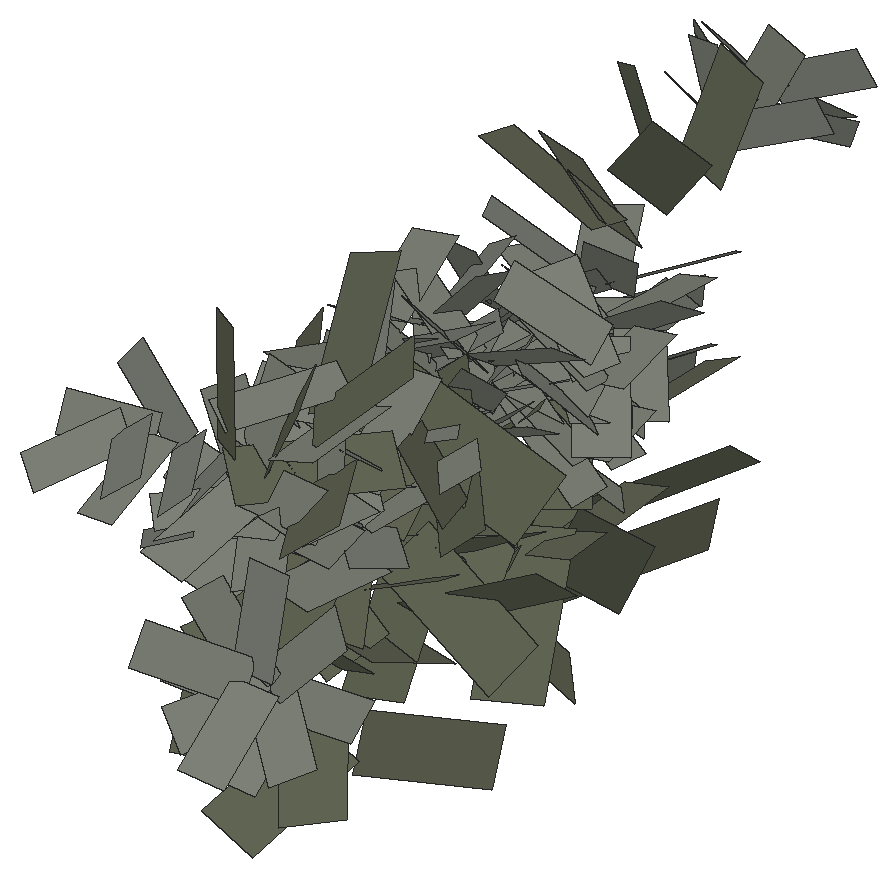
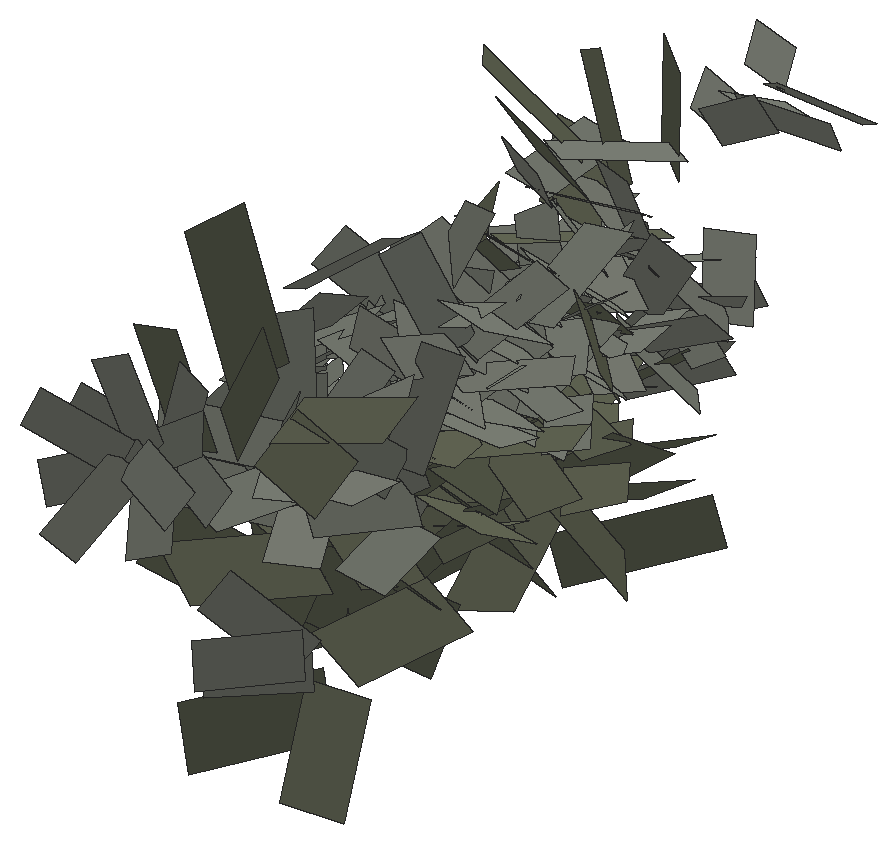
# SketchUp Ruby script. Lengths in inches.
U = 1.inch
M = Sketchup.active_model
def pt(a) = Geom::Point3d.new(a.map { |v| v * U })
def face(e, loops, mat)
  f = e.add_face(loops[0].map { |a| pt(a) })
  loops[1..].each { |l| e.add_face(l.map { |a| pt(a) }).erase! }
  f.material = f.back_material = mat if mat
  f
end
# faces: each face lists its corners as indices into pts; further lists are holes
def faces(e, pts, list, mat = nil) = list.each { |f| face(e, (f[0].is_a?(Array) ? f : [f]).map { |l| l.map { |i| pts[i] } }, mat) }
# xy, xz, yz: faces in a plane at the given z, y or x. An outline is a flat list of corners, or four numbers for a rectangle; further outlines are holes
def ring(l) = l.size == 4 ? [[l[0], l[1]], [l[2], l[1]], [l[2], l[3]], [l[0], l[3]]] : l.each_slice(2).to_a
def flat(e, list, mat, &to3) = list.each { |f| face(e, (f[0].is_a?(Array) ? f : [f]).map { |l| ring(l).map { |u, v| to3.(u, v) } }, mat) }
def xy(e, z, list, mat = nil) = flat(e, list, mat) { |x, y| [x, y, z] }
def xz(e, y, list, mat = nil) = flat(e, list, mat) { |x, z| [x, y, z] }
def yz(e, x, list, mat = nil) = flat(e, list, mat) { |y, z| [x, y, z] }
def lines(e, pts, list) = list.each { |a, b| e.add_line(pt(pts[a]), pt(pts[b])) }
# prism: a flat outline (further loops are holes) pulled along v
def prism(e, loops, v, mat = nil)
  f = face(e, loops, mat); d = Geom::Vector3d.new(v.map { |x| x * U })
  f.pushpull(f.normal.samedirection?(d) ? d.length : -d.length)
end
def box(e, o, s, mat = nil) = prism(e, [[o, [o[0] + s[0], o[1], o[2]], [o[0] + s[0], o[1] + s[1], o[2]], [o[0], o[1] + s[1], o[2]]]], [0, 0, s[2]], mat)
def at(x, y, z, deg = 0) = Geom::Transformation.translation(pt([x, y, z])) * Geom::Transformation.rotation(ORIGIN, Z_AXIS, deg.degrees)
def axes(o, x, y, z) = Geom::Transformation.new([*x, 0, *y, 0, *z, 0, *pt(o).to_a, 1])
def part(name) = M.definitions.add(name)
# library, detail: a bought-in or finely detailed component or shape, given as its bounding box
def library(name, o, s) = part(name).tap { |d| box(d.entities, o, s) }
def detail(e, o, s) = box(e.add_group.entities, o, s)
def put(e, d, t, mat = nil) = e.add_instance(d, t).tap { |i| i.material = mat if mat }
def group(e, t, mat = nil) = e.add_group.tap { |g| g.transformation = t; g.material = mat if mat }.entities
root = M.entities
M.materials.add("viburnumblaasdfas0df1w06d").color = [98, 102, 84]
M.materials.add("viburnumbladsadfasdfad0w122").color = [125, 129, 119]
c1 = part("Component\#315")
p = [[0.25,0,0],[2.05,0.01,0.35],[1.81,4.2,1.66],[0,4.19,1.3125]]
faces(c1.entities,p,[[0,1,2,3]],"viburnumbladsadfasdfad0w122")
c2 = part("viburnumblad2")
put(c2.entities,c1,axes([-19.23,-4.49,-32.18],[83.35428,0,0],[0,79.38502,0],[0,0,83.35428]))
c3 = part("Component\#314")
p = [[0.14,0,0],[2.58,0.05,0.25],[2.44,5.11,2.64],[0,5.05,2.39]]
faces(c3.entities,p,[[0,1,2,3]],"viburnumblaasdfas0df1w06d")
c4 = part("viburnumblad1\#2")
put(c4.entities,c3,axes([-37.25,6.23,19.31],[75.98784,0,0],[0,65.50676,0],[0,0,75.98784]))
put(root,c2,axes([2206.24,252.28,28.43],[-0.00034,0.00733,0.00907],[-0.01154,0.00172,-0.00184],[-0.00225,-0.00876,0.00608]))
put(root,c4,axes([2207.27,278.16,26.82],[-0.00128,0.01292,-0.00526],[-0.01614,-0.0018,-0.00049],[-0.00098,0.00473,0.0118]))
put(root,c2,axes([2206.21,259.38,21.66],[0.00219,0.00955,0.00743],[-0.01307,0.00092,0.00265],[0.0015,-0.00837,0.01031]))
put(root,c4,axes([2205.43,261.88,20.89],[0.01183,-0.00442,0.01203],[-0.00182,0.01827,0.0085],[-0.01272,-0.00605,0.01028]))
put(root,c2,axes([2202.79,283.42,19.07],[0.00504,-0.005,0.01036],[0.00925,0.00849,-0.00041],[-0.00684,0.0078,0.00709]))
put(root,c2,axes([2206.37,251.14,29.41],[-0.00814,0.00715,0.0046],[-0.00805,-0.00423,-0.00746],[-0.00268,-0.00803,0.00677]))
put(root,c2,axes([2204.18,267.51,21.67],[-0.01,-0.00652,-0.00001],[0.00542,-0.00831,-0.00274],[0.00166,-0.00256,0.01102]))
put(root,c2,axes([2202.71,257.99,22.83],[0.00888,-0.0091,-0.0009],[0.00823,0.00741,0.00631],[-0.00398,-0.00497,0.01104]))
put(root,c2,axes([2203.77,274.18,21],[0.0138,0.00142,0.00148],[-0.00058,0.0109,-0.00504],[-0.00186,0.00548,0.01205]))
put(root,c2,axes([2205.47,275.59,24.34],[-0.01322,-0.00136,-0.00142],[0.00017,-0.01043,0.00835],[-0.00196,0.00824,0.01034]))
put(root,c4,axes([2207.03,278.73,26.75],[0.00337,0.00858,-0.01052],[-0.01574,0.00327,-0.00237],[0.0008,0.00999,0.00793]))
put(root,c2,axes([2205.18,262.88,23.52],[-0.01211,-0.00173,0.00211],[0.00069,-0.01077,-0.00395],[0.00303,-0.00413,0.011]))
put(root,c2,axes([2206.93,269.17,25.19],[-0.0062,0.01038,-0.0034],[-0.01088,-0.00717,-0.00204],[-0.00346,0.00185,0.01194]))
put(root,c4,axes([2205.48,276.63,14.54],[0.01075,0.00741,0.00439],[-0.00265,0.0107,-0.01157],[-0.00831,0.00706,0.00843]))
put(root,c2,axes([2203.84,267.17,26.41],[0.01523,-0.00004,0.00037],[-0.00005,0.01486,0.00338],[-0.00037,-0.00338,0.01485]))
put(root,c2,axes([2206.5,269,23.43],[0.0027,0.01283,-0.00001],[-0.01066,0.00224,-0.00301],[-0.00327,0.0007,0.01211]))
put(root,c2,axes([2205.36,258.77,23.13],[0.01106,0.0052,0.00541],[-0.00756,0.007,0.00872],[0.00055,-0.01018,0.00865]))
put(root,c2,axes([2204.26,257.63,23.09],[-0.00865,-0.00796,-0.00491],[0.00846,-0.00952,0.00054],[-0.00401,-0.0029,0.01175]))
put(root,c2,axes([2202.83,267.875,22.0625],[0.00554,-0.00849,-0.00419],[0.01058,0.00621,0.0014],[0.00119,-0.0044,0.01049]))
put(root,c2,axes([2203.29,258.99,20],[0.00852,-0.00783,-0.00192],[0.00823,0.00741,0.00631],[-0.003,-0.00593,0.01088]))
put(root,c2,axes([2205.58,269.34,24.61],[0.00987,0.007,0.00339],[-0.00618,0.00957,-0.0018],[-0.0039,-0.00027,0.01194]))
put(root,c4,axes([2208.25,268.6,20.74],[-0.00473,0.01294,-0.00003],[-0.01473,-0.00539,-0.00308],[-0.0025,-0.00088,0.01352]))
put(root,c2,axes([2207.21,258.51,22.89],[-0.00749,0.00812,0.00752],[-0.01012,-0.00577,-0.00385],[0.00099,-0.00855,0.01022]))
put(root,c2,axes([2206.23,253.68,27.9],[0.00736,0.00309,0.0079],[-0.00921,0.00654,0.0057],[-0.00262,-0.00929,0.00521]))
put(root,c4,axes([2203.95,266.08,17.85],[-0.0111,-0.00766,0.00199],[0.00742,-0.01279,-0.00569],[0.00489,-0.00308,0.01206]))
put(root,c2,axes([2203.05,263.78,22.82],[0.00848,-0.00639,-0.00524],[0.0093,0.00903,0.00402],[0.00207,-0.0066,0.01002]))
put(root,c2,axes([2204.25,267.21,22.59],[0.01462,-0.00004,0.00036],[-0.00005,0.01605,0.00365],[-0.00037,-0.00338,0.01485]))
put(root,c2,axes([2204.8125,266.82,24.35],[-0.00958,-0.00624,-0.00001],[0.00602,-0.00923,-0.00305],[0.00166,-0.00256,0.01102]))
put(root,c4,axes([2204.25,271.81,15.78],[0.01294,-0.00163,0.0067],[0.00488,0.01526,-0.00571],[-0.00546,0.00626,0.01208]))
put(root,c2,axes([2206.84,287.89,29.93],[0.00367,0.00526,-0.00978],[-0.01118,0.00267,-0.00269],[0.001,0.0097,0.00482]))
put(root,c4,axes([2207.83,268.4,18.21],[0.00606,0.01155,0.00446],[-0.01316,0.00831,-0.00362],[-0.00493,-0.00229,0.01266]))
put(root,c2,axes([2204.25,282.65,18.33],[-0.00352,-0.00882,0.00823],[0.00998,0.00284,0.00731],[-0.00692,0.00849,0.00615]))
put(root,c2,axes([2206.95,285.46,28.96],[0.00325,0.00384,-0.00943],[-0.01118,0.00267,-0.00269],[0.00139,0.01021,0.00373]))
put(root,c2,axes([2206.84,269.7,26.86],[-0.01136,0.00239,-0.0048],[-0.00314,-0.01208,0.00143],[-0.00434,0.00249,0.01152]))
put(root,c2,axes([2204.6,263.86,22.52],[-0.00866,-0.0095,-0.00259],[0.00823,-0.00655,-0.00374],[0.002,-0.00468,0.01099]))
put(root,c2,axes([2207.41,276.27,23.98],[0.0037,0.01302,-0.00469],[-0.01381,0.00379,-0.00038],[0.0009,0.00462,0.01353]))
put(root,c2,axes([2206.52,266.7,26.43],[-0.01523,0.00004,-0.00037],[-0.00005,-0.01523,0.00032],[-0.00037,0.00032,0.01523]))
put(root,c4,axes([2203.32,268.9,19.23],[-0.00529,-0.01137,-0.00003],[0.01295,-0.00601,-0.0028],[0.00218,-0.00104,0.01231]))
put(root,c2,axes([2203.68,275.4,22.09],[0.00964,-0.00707,0.00598],[0.00804,0.00897,-0.00235],[-0.00301,0.00576,0.01168]))
put(root,c2,axes([2203.52,267.28,24.8],[0.00577,-0.00885,-0.00437],[0.0098,0.00575,0.0013],[0.00119,-0.0044,0.01049]))
put(root,c2,axes([2203.8,267.68,23.28],[-0.00269,-0.01067,-0.0031],[0.01162,-0.00239,-0.00186],[0.00104,-0.00341,0.01086]))
put(root,c4,axes([2207.89,261.97,15.1],[0.00636,0.01278,0.00656],[-0.01653,0.00548,0.00535],[0.00178,-0.00782,0.01351]))
put(root,c2,axes([2203.82,258.79,21.62],[0.00016,-0.01206,-0.00411],[0.01207,-0.0013,0.00429],[-0.00443,-0.00391,0.01129]))
put(root,c2,axes([2208.1,276.89,25.73],[-0.00715,0.01146,-0.00475],[-0.01239,-0.00628,0.0035],[0.00072,0.00585,0.01305]))
put(root,c2,axes([2204.05,281.32,17.3125],[0.00529,-0.00535,0.00878],[0.00925,0.00849,-0.00041],[-0.00626,0.00721,0.00817]))
put(root,c2,axes([2206.74,267.15,22.81],[-0.01389,0,-0.00185],[-0.00005,-0.01523,0.00032],[-0.00201,0.00032,0.0151]))
put(root,c2,axes([2204.92,270.49,26.02],[0.01136,-0.00239,0.0048],[0.002,0.01232,0.0014],[-0.00498,-0.0005,0.01153]))
put(root,c2,axes([2203.82,262.74,25.59],[0.00883,-0.00666,-0.00546],[0.00861,0.00836,0.00373],[0.00207,-0.0066,0.01002]))
put(root,c2,axes([2207.31,261.64,23.91],[0.00207,0.01081,-0.00198],[-0.01024,0.00263,0.00364],[0.00398,0.00114,0.01039]))
put(root,c4,axes([2207.83,263.29,17.43],[-0.01218,0.00376,0.00725],[-0.00872,-0.0119,-0.00846],[0.0032,-0.00977,0.01045]))
put(root,c2,axes([2207.85,286.6,29.39],[-0.00534,0.00476,-0.00922],[-0.00963,-0.00133,0.0047],[0.00092,0.0102,0.00386]))
put(root,c4,axes([2208.4,261.46,11.49],[-0.00011,0.00616,0.01357],[-0.0165,-0.00475,0.00202],[0.00445,-0.01294,0.00591]))
put(root,c4,axes([2204.5625,262.1,12.5],[0.01021,-0.01095,0.0021],[0.01009,0.01114,0.00903],[-0.00698,-0.00405,0.01279]))
put(root,c2,axes([2206.27,286.84,28.9375],[0.01052,0.00268,-0.00462],[-0.0054,0.00599,-0.0087],[0.00028,0.0093,0.00555]))
put(root,c2,axes([2206.46,277.57,25.375],[0.01238,0.00695,-0.00189],[-0.0072,0.01199,-0.00308],[0.00008,0.00361,0.01386]))
put(root,c4,axes([2203.39,265.61,20.18],[-0.00229,-0.01326,-0.00295],[0.0155,-0.0021,-0.00237],[0.00206,-0.00324,0.01267]))
put(root,c2,axes([2207.49,259.9,22.07],[-0.0137,0.00216,0.00156],[-0.00229,-0.00943,-0.00711],[-0.00005,-0.00804,0.01068]))
put(root,c2,axes([2204.07,263.57,24.15],[0.00038,-0.01114,-0.00561],[0.01301,0.00109,-0.00087],[0.0016,-0.0057,0.01058]))
put(root,c2,axes([2208.21,268.07,23.86],[-0.00604,0.00926,-0.00001],[-0.00892,-0.00582,-0.00295],[-0.00247,-0.0016,0.01066]))
put(root,c2,axes([2206.62,261.9,22.62],[0.00864,0.00566,-0.00294],[-0.00615,0.01026,0.00169],[0.00342,0.0003,0.01064]))
put(root,c2,axes([2207.61,257.72,24.57],[-0.01312,0.00207,0.00149],[-0.00255,-0.01047,-0.0079],[-0.00005,-0.00804,0.01068]))
put(root,c2,axes([2205.34,262.71,25.21],[-0.00829,-0.0091,-0.00248],[0.00914,-0.00728,-0.00415],[0.002,-0.00468,0.01099]))
put(root,c2,axes([2205.54,275.61,22.32],[-0.00906,-0.00899,0.00397],[0.00943,-0.00624,0.00738],[-0.00308,0.00772,0.01046]))
put(root,c2,axes([2206.97,268.62,23.55],[0.00856,0.00558,0.00422],[-0.00642,0.00891,0.00123],[-0.00278,-0.00341,0.01014]))
put(root,c2,axes([2207.84,269.77,23.85],[-0.01091,0.00229,-0.00461],[-0.00339,-0.01305,0.00154],[-0.00434,0.00249,0.01152]))
put(root,c2,axes([2204.46,276.67,23.51],[0.00041,-0.01136,0.00703],[0.01289,0.00219,0.00278],[-0.00352,0.00669,0.01102]))
put(root,c2,axes([2207.37,252.56,29.38],[-0.01118,0.00278,-0.00257],[-0.00011,-0.00839,-0.00838],[-0.00365,-0.00753,0.00688]))
put(root,c4,axes([2208.38,281.04,27.26],[-0.00982,0.00575,-0.00616],[-0.00925,-0.00382,0.01097],[0.00277,0.01054,0.00496]))
put(root,c2,axes([2208.1,268.31,22.32],[0.00178,0.0105,0.00298],[-0.0098,0.00211,-0.00159],[-0.00226,-0.0026,0.01051]))
put(root,c2,axes([2208.25,261.8125,25.13],[-0.00607,0.00939,0.00026],[-0.0086,-0.00567,0.00435],[0.00378,0.00216,0.0103]))
put(root,c2,axes([2208.47,267.01,23.85],[0.00229,0.01091,-0.00461],[-0.01305,0.00339,0.00154],[0.00249,0.00434,0.01152]))
put(root,c2,axes([2207.08,276.19,22.09],[0.01189,0.00667,-0.00181],[-0.00777,0.01295,-0.00333],[0.00008,0.00361,0.01386]))
put(root,c2,axes([2205.38,258.375,25.11],[0.01312,-0.00207,-0.00149],[0.00246,0.00822,0.01025],[-0.00067,-0.01033,0.00845]))
put(root,c2,axes([2208.39,268.01,26.86],[0.00239,0.01136,-0.0048],[-0.01208,0.00314,0.00143],[0.00249,0.00434,0.01152]))
put(root,c2,axes([2206.97,262.35,25.38],[0.009,0.00589,-0.00306],[-0.00569,0.0095,0.00156],[0.00342,0.0003,0.01064]))
put(root,c2,axes([2208.15,285.61,28.56],[-0.01171,0.00153,-0.0034],[-0.00332,-0.0036,0.00923],[0.00008,0.01052,0.00323]))
put(root,c2,axes([2205.93,270.21,23.2],[0.01089,-0.00213,0.00325],[0.002,0.01232,0.0014],[-0.00372,-0.00076,0.01198]))
put(root,c2,axes([2204.85,275.1,20.74],[0.00073,-0.01105,0.00534],[0.01289,0.00219,0.00278],[-0.00345,0.00543,0.01171]))
put(root,c2,axes([2204.4375,267.96,24.53],[0.01077,-0.01075,-0.00083],[0.01118,0.01095,0.00335],[-0.00168,-0.00283,0.01488]))
put(root,c4,axes([2209.54,261.56,17.48],[-0.00702,0.01204,0.00725],[-0.01547,-0.00958,0.00093],[0.00442,-0.0058,0.01392]))
put(root,c4,axes([2207.29,266.6,20.74],[0.01294,0.00473,-0.00003],[-0.00539,0.01473,-0.00308],[-0.00088,0.0025,0.01352]))
put(root,c2,axes([2206.23,268.1,24.57],[-0.01077,-0.01069,-0.00135],[0.00977,-0.00996,0.00094],[-0.00168,-0.00022,0.01514]))
put(root,c4,axes([2206.81,256.54,27.22],[0.01089,-0.00679,0.00142],[0.00218,0.00667,0.0129],[-0.00665,-0.00902,0.00468]))
put(root,c2,axes([2208.88,268.68,21.27],[-0.0063,0.00967,-0.00001],[-0.00803,-0.00524,-0.00265],[-0.00247,-0.0016,0.01066]))
put(root,c2,axes([2206.57,251.99,30.59],[-0.00766,-0.00322,-0.00823],[0.00764,-0.00813,-0.00386],[-0.0046,-0.00755,0.00633]))
put(root,c2,axes([2209.0625,260.6,21.01],[0.00051,0.01437,0.00412],[-0.01266,-0.00025,0.00242],[0.00266,-0.00396,0.0135]))
put(root,c2,axes([2209.23,267.52,25.26],[-0.007,0.00987,-0.00339],[-0.01018,-0.00558,0.00479],[0.00226,0.00542,0.01111]))
put(root,c2,axes([2207.77,269.08,21.07],[0.0081,0.00545,0.00286],[-0.00642,0.00891,0.00123],[-0.00184,-0.00279,0.01054]))
put(root,c4,axes([2206.66,264.22,12.74],[0.01682,-0.00022,0.00237],[-0.00091,0.01794,0.00812],[-0.00224,-0.00704,0.0153]))
put(root,c2,axes([2209.5,259.43,24.33],[0.00048,0.01376,0.00394],[-0.01406,-0.00028,0.00269],[0.00266,-0.00396,0.0135]))
put(root,c4,axes([2210.08,269.14,16.68],[-0.00341,0.01096,0.00392],[-0.01337,-0.00302,-0.00319],[-0.00164,-0.0045,0.01114]))
put(root,c2,axes([2207.33,270.53,25.26],[-0.00987,-0.007,-0.00339],[0.00558,-0.01018,0.00479],[-0.00542,0.00226,0.01111]))
put(root,c2,axes([2207.86,267.92,25.19],[0.01038,0.0062,-0.0034],[-0.00717,0.01088,-0.00204],[0.00185,0.00346,0.01194]))
put(root,c2,axes([2209.72,260.02,27.65],[-0.00274,0.01284,0.00559],[-0.01166,-0.00082,-0.00384],[-0.00348,-0.00589,0.01184]))
put(root,c4,axes([2207.95,268.23,13.125],[-0.01776,-0.00139,0.00308],[0.00179,-0.02087,0.00087],[0.003,0.001,0.0178]))
put(root,c2,axes([2209.12,276.93,23.82],[-0.01381,0.0032,-0.00202],[-0.0038,-0.01243,0.00635],[-0.00034,0.00659,0.01271]))
put(root,c4,axes([2205.85,262.61,19.81],[0.01107,-0.00525,0.00049],[0.00612,0.01279,-0.0012],[0,0.00115,0.01221]))
put(root,c2,axes([2206.28,271.14,26.51],[-0.00259,-0.01229,0.00001],[0.0107,-0.00225,0.00618],[-0.00604,0.00128,0.01094]))
put(root,c2,axes([2205.9375,271.07,24.65],[0.0062,-0.01038,0.0034],[0.00931,0.00714,0.00482],[-0.00586,0.00014,0.01111]))
put(root,c2,axes([2208.5625,262.2,23.52],[-0.01065,0.00247,0.00234],[-0.00174,-0.01065,0.00331],[0.00294,0.00276,0.01043]))
put(root,c2,axes([2206.4,288.54,28.68],[0.01122,-0.00147,0.00326],[0.00359,0.00643,-0.00917],[-0.00081,0.00924,0.00561]))
put(root,c2,axes([2209.58,255.5,16.85],[-0.00011,0.00779,0.00854],[-0.01208,-0.00262,0.00224],[0.00345,-0.0089,0.00816]))
put(root,c4,axes([2209.54,270.13,14.24],[0.00865,0.00658,0.00734],[-0.00992,0.01145,0.00143],[-0.0049,-0.0056,0.0108]))
put(root,c2,axes([2205.41,268.27,26.5625],[0,-0.01516,-0.00154],[0.01507,-0.00022,0.00221],[-0.00223,-0.00152,0.015]))
put(root,c2,axes([2205.73,268.45,22.8],[0,-0.01583,-0.00161],[0.01357,-0.0002,0.00199],[-0.00223,-0.00152,0.015]))
put(root,c2,axes([2209.04,269.05,22.82],[-0.01032,0.0026,-0.00299],[-0.00231,-0.01123,-0.0018],[-0.0033,-0.001,0.0105]))
put(root,c2,axes([2207.39,259.62,23.99],[-0.01106,-0.0052,-0.00541],[0.00776,-0.00965,-0.0066],[-0.00127,-0.0082,0.01048]))
put(root,c4,axes([2205.0625,268.87,18.96],[0.0081,-0.01447,0.00211],[0.01627,0.00971,0.00411],[-0.00412,0.00005,0.0162]))
put(root,c2,axes([2206.71,262.75,23.89],[0.01065,-0.00247,-0.00234],[0.00251,0.01145,-0.00069],[0.00243,0.00013,0.01091]))
put(root,c2,axes([2210.1,259.58,29.55],[-0.01065,0.00857,-0.00023],[-0.00787,-0.00997,-0.00669],[-0.00415,-0.00484,0.01209]))
put(root,c4,axes([2211.27,262.26,22.42],[0.00121,0.01104,0.01007],[-0.01675,0.00403,-0.00241],[-0.00386,-0.00953,0.01091]))
put(root,c2,axes([2207.24,269.62,22.34],[0.01032,-0.0026,0.00299],[0.00135,0.01024,0.00424],[-0.00373,-0.00356,0.00978]))
put(root,c2,axes([2208.67,260.29,22.69],[0.01044,0.00958,0.00206],[-0.00879,0.00856,0.00474],[0.00211,-0.00514,0.0132]))
put(root,c2,axes([2210.35,260.39,22.625],[-0.00976,0.00988,0.00351],[-0.01076,-0.01049,-0.00039],[0.00219,-0.00277,0.01388]))
put(root,c2,axes([2207.46,254.09,29.29],[-0.00655,-0.0022,-0.00816],[0.00764,-0.00813,-0.00386],[-0.0054,-0.00785,0.00541]))
put(root,c4,axes([2207.74,262.7,20.09],[-0.01365,-0.00518,-0.0014],[0.0059,-0.01311,-0.00908],[0.00168,-0.00777,0.01232]))
put(root,c2,axes([2205.93,259.92,24.27],[0.00749,-0.00812,-0.00752],[0.01093,0.00403,0.00654],[-0.00171,-0.00982,0.0089]))
put(root,c4,axes([2208.21,269.64,15.44],[0.01224,-0.00166,0.00834],[0.00122,0.01717,0.00163],[-0.00844,-0.00056,0.01227]))
put(root,c2,axes([2209.99,253.16,18.7],[0.00026,0.00745,0.01011],[-0.01208,-0.00262,0.00224],[0.00344,-0.00977,0.00711]))
put(root,c2,axes([2206.73,277.62,23.4],[0.01381,-0.0032,0.00202],[0.00375,0.01421,-0.00318],[-0.00124,0.00342,0.01385]))
put(root,c2,axes([2208.97,254.51,18.08],[0.00896,0.00627,0.00619],[-0.00837,0.00305,0.00903],[0.00298,-0.01046,0.00629]))
put(root,c2,axes([2208.18,287.24,28.21],[-0.01052,-0.00268,0.00462],[0.00552,-0.00368,0.01018],[-0.00102,0.01046,0.0033]))
put(root,c4,axes([2210.63,267.97,12.74],[0.00022,0.01682,0.00237],[-0.01794,-0.00091,0.00812],[0.00704,-0.00224,0.0153]))
put(root,c4,axes([2210.22,269.52,18.9],[-0.011,0.00511,-0.00003],[-0.00581,-0.01252,-0.00271],[-0.00101,-0.0021,0.0119]))
put(root,c4,axes([2208.45,283.35,26.95],[-0.01249,0.00074,0.00321],[0.00342,-0.00484,0.01344],[0.00175,0.01171,0.00271]))
put(root,c4,axes([2205.97,271.38,13.05],[0.00095,-0.01143,0.01095],[0.01752,0.00456,0.00324],[-0.00472,0.01026,0.01113]))
put(root,c4,axes([2207.3,275.96,12.18],[0.00521,-0.00318,0.0136],[0.01189,0.01244,-0.00164],[-0.00949,0.00985,0.00593]))
put(root,c4,axes([2210.57,272.14,16.32],[-0.00358,0.0126,0.00711],[-0.01496,-0.00708,0.005],[0.00656,-0.00511,0.01237]))
put(root,c4,axes([2206.93,262.36,15.14],[-0.00936,-0.00715,0.0061],[0.00985,-0.01174,0.00135],[0.00403,0.00472,0.01172]))
put(root,c4,axes([2211.625,261.5,25.09],[-0.01024,0.01003,0.00441],[-0.01249,-0.0094,-0.00763],[-0.00202,-0.00765,0.01274]))
put(root,c2,axes([2208.13,262.86,22.23],[-0.00842,-0.00565,0.00174],[0.00635,-0.00914,0.00106],[0.00096,0.00194,0.01097]))
put(root,c4,axes([2208.52,259.95,27.32],[0.01421,-0.00084,0.00442],[-0.0012,0.01582,0.00687],[-0.00438,-0.00595,0.01294]))
put(root,c2,axes([2209.83,268.57,26.51],[-0.01229,0.00259,0.00001],[-0.00225,-0.0107,0.00618],[0.00128,0.00604,0.01094]))
put(root,c2,axes([2206.66,261.01,23.05],[-0.00242,-0.00904,-0.00878],[0.01402,-0.00344,-0.00033],[-0.00196,-0.00893,0.00974]))
put(root,c2,axes([2208.64,261,27.8125],[0.01184,0.00091,0.00415],[-0.00322,0.01148,0.00668],[-0.0033,-0.00735,0.01104]))
put(root,c2,axes([2206.92,258.85,25.62],[-0.00252,-0.00942,-0.00914],[0.01298,-0.00318,-0.00031],[-0.00196,-0.00893,0.00974]))
put(root,c2,axes([2207,263.25,22.375],[0.00633,-0.0098,-0.00027],[0.00833,0.00542,-0.00155],[0.00159,0.00072,0.01104]))
put(root,c2,axes([2208.66,269.32,24.29],[-0.00856,-0.00558,-0.00422],[0.00556,-0.00947,0.00126],[-0.00425,-0.00115,0.01014]))
put(root,c4,axes([2206.18,263.17,17.63],[0.00308,-0.0114,0.00333],[0.01375,0.00318,-0.00182],[0.00071,0.00361,0.0117]))
put(root,c2,axes([2206.95,287.48,27.76],[0.00534,-0.00476,0.00922],[0.0104,0.00387,-0.00404],[-0.00165,0.00955,0.00498]))
put(root,c2,axes([2207.69,268.35,23.43],[0.01283,-0.0027,-0.00001],[0.00224,0.01066,-0.00301],[0.0007,0.00327,0.01211]))
put(root,c4,axes([2207.25,276.23,18.27],[0.01313,-0.00582,0.00636],[0.00841,0.01593,-0.00278],[-0.00467,0.00494,0.01417]))
put(root,c2,axes([2207.41,269.87,23.98],[0.00604,-0.00926,0.00001],[0.00806,0.00526,0.00544],[-0.00456,-0.00296,0.00963]))
put(root,c4,axes([2207.1,267.02,18.21],[0.01155,-0.00606,0.00446],[0.00831,0.01316,-0.00362],[-0.00229,0.00493,0.01266]))
put(root,c2,axes([2210.72,254.74,17.86],[-0.00859,0.00427,0.00811],[-0.00794,-0.00683,-0.00482],[0.00302,-0.00917,0.00803]))
put(root,c2,axes([2207.74,269.37,26.37],[0.01229,-0.00259,-0.00001],[0.00249,0.01185,-0.00335],[0.0007,0.00327,0.01211]))
put(root,c4,axes([2210.09,260.1,13.64],[-0.01186,-0.00066,0.00699],[-0.00532,-0.01121,-0.01007],[0.00532,-0.0098,0.0081]))
put(root,c2,axes([2208.85,278.44,25.1875],[-0.01238,-0.00695,0.00189],[0.007,-0.01076,0.00634],[-0.00166,0.00641,0.0127]))
put(root,c2,axes([2208.16,261.75,21.51],[0.01298,0.00037,-0.00224],[0.00059,0.01317,0.00559],[0.0024,-0.0056,0.01296]))
put(root,c2,axes([2207.59,286.2,27.32],[-0.00352,-0.00505,0.00939],[0.01197,-0.00026,0.00408],[-0.00173,0.01006,0.00403]))
put(root,c2,axes([2207.7,263.53,23.52],[-0.00207,-0.01081,0.00198],[0.01001,-0.00209,-0.00093],[0.00139,0.00174,0.01096]))
put(root,c2,axes([2208.73,263.11,24.83],[-0.009,-0.00589,0.00306],[0.00635,-0.00914,0.00106],[0.00195,0.00259,0.0107]))
put(root,c4,axes([2206.71,269.47,16.39],[-0.00613,-0.01546,0.00166],[0.01796,-0.00686,0.00247],[-0.00138,0.00232,0.01649]))
put(root,c2,axes([2207.82,288.77,28.31],[-0.00367,-0.00526,0.00978],[0.01109,-0.00025,0.00378],[-0.00173,0.01006,0.00403]))
put(root,c2,axes([2209.11,277.35,21.94],[-0.01116,-0.00699,0.00046],[0.007,-0.01076,0.00634],[-0.00299,0.00562,0.01283]))
put(root,c2,axes([2207.45,263.65,25.08],[0.00607,-0.00939,-0.00026],[0.00926,0.00603,-0.00173],[0.00159,0.00072,0.01104]))
put(root,c2,axes([2209.23,269.99,21.65],[-0.00821,-0.00536,-0.00406],[0.00601,-0.01023,0.00136],[-0.00425,-0.00115,0.01014]))
put(root,c2,axes([2210.49,261.72,21.19],[-0.01371,0.0002,0.00098],[-0.0004,-0.01527,-0.00242],[0.00098,-0.00226,0.01411]))
put(root,c2,axes([2207.21,279.12,24.83],[0.00715,-0.01146,0.00475],[0.01219,0.00751,-0.00024],[-0.0023,0.00416,0.01351]))
put(root,c2,axes([2208.51,260.87,24.8125],[0.01428,-0.00021,-0.00102],[0.00059,0.01317,0.00559],[0.00086,-0.00561,0.01315]))
put(root,c4,axes([2208.0625,258.51,27.16],[0.00428,-0.01029,-0.00658],[0.01194,-0.00078,0.00879],[-0.00649,-0.00737,0.00685]))
put(root,c2,axes([2208.4375,270.15,22.88],[-0.00178,-0.0105,-0.00298],[0.00981,-0.00286,0.00422],[-0.00478,-0.00196,0.00978]))
put(root,c2,axes([2208.11,278.53,23.11],[-0.0037,-0.01302,0.00469],[0.0125,-0.00235,0.00334],[-0.00247,0.0054,0.01303]))
put(root,c2,axes([2210.64,256.1875,17.35],[-0.01296,-0.00148,0.00142],[-0.00002,-0.00776,-0.00823],[0.00196,-0.00903,0.00851]))
put(root,c4,axes([2211.09,264.73,20.21],[0.01304,-0.00033,0.00964],[-0.00605,0.01553,0.00873],[-0.00811,-0.00915,0.01066]))
put(root,c2,axes([2207.69,277.82,21.5625],[0.00747,-0.01197,0.00496],[0.01097,0.00676,-0.00022],[-0.0023,0.00416,0.01351]))
put(root,c2,axes([2208.03,269.27,24.61],[0.007,-0.00987,0.00339],[0.00957,0.00618,-0.0018],[-0.00027,0.0039,0.01194]))
put(root,c2,axes([2211.01,260.41,24.51],[-0.01428,0.00021,0.00102],[-0.00037,-0.01414,-0.00224],[0.00098,-0.00226,0.01411]))
put(root,c4,axes([2208.75,279.61,27.58],[-0.01185,-0.00554,0.00715],[0.01005,-0.01197,0.00738],[0.00259,0.00922,0.01142]))
put(root,c2,axes([2209.11,253.82,19.84],[0.01241,0.00141,-0.00136],[0.00049,0.00618,0.01093],[0.0019,-0.01085,0.00605]))
put(root,c2,axes([2210.73,261.07,28.6],[-0.01194,-0.00018,-0.00545],[0.00215,-0.01397,-0.00426],[-0.00531,-0.00441,0.0118]))
put(root,c2,axes([2212.04,273.14,21.15],[0.00007,0.01222,-0.00309],[-0.01226,0.00091,0.00331],[0.0034,0.00296,0.01177]))
put(root,c2,axes([2209.76,268.91,24.65],[-0.01038,-0.0062,0.0034],[0.00714,-0.00931,0.00482],[0.00014,0.00586,0.01111]))
put(root,c4,axes([2211.29,269.45,20.05],[0.00989,0.00806,-0.00127],[-0.00946,0.01134,-0.00169],[0.00005,0.00193,0.01267]))
put(root,c4,axes([2212.09,270.61,11.87],[-0.01033,0.0106,0.00208],[-0.0106,-0.01173,0.00714],[0.00578,0.00298,0.01347]))
put(root,c2,axes([2212.37,271.09,24.15],[-0.00324,0.01089,0.00211],[-0.01127,-0.00408,0.00376],[0.00428,-0.00101,0.01177]))
put(root,c2,axes([2211.29,253.84,19.29],[-0.01241,-0.00141,0.00136],[-0.00002,-0.00862,-0.00914],[0.00196,-0.00903,0.00851]))
put(root,c2,axes([2212.55,270.17,22.8125],[-0.00179,0.01029,-0.00409],[-0.01223,-0.00094,0.00298],[0.00221,0.00457,0.01052]))
put(root,c2,axes([2212.54,271.02,25.63],[-0.00186,0.01072,-0.00426],[-0.01132,-0.00087,0.00276],[0.00221,0.00457,0.01052]))
put(root,c4,axes([2212.54,265.56,14.61],[0.0025,0.01316,0.00583],[-0.01545,-0.00015,0.00696],[0.00546,-0.00635,0.01198]))
put(root,c2,axes([2208.9,268.92,23.2],[-0.00213,-0.01089,0.00325],[0.01232,-0.002,0.0014],[-0.00076,0.00372,0.01198]))
put(root,c4,axes([2210.52,267.16,12.65],[0.01503,0.00487,0.00033],[-0.00521,0.01551,0.00826],[0.00191,-0.00687,0.0141]))
put(root,c2,axes([2211.85,270.89,25.74],[0.00616,0.01091,0.00086],[-0.01009,0.00525,0.00563],[0.00448,-0.00342,0.01123]))
put(root,c4,axes([2212.97,266.74,20.89],[0.00442,0.01183,0.01203],[-0.01827,-0.00182,0.0085],[0.00605,-0.01272,0.01028]))
put(root,c2,axes([2211.48,274.17,22.65],[0.00886,0.00826,-0.00347],[-0.00846,0.00932,0.00058],[0.00295,0.00192,0.0121]))
put(root,c2,axes([2212.69,273.08,19.59],[-0.0083,0.00785,-0.00197],[-0.00857,-0.00783,0.00492],[0.002,0.00498,0.01141]))
put(root,c2,axes([2211.91,270.78,24.15],[0.00682,0.00858,-0.00405],[-0.00975,0.00742,-0.00069],[0.00196,0.0036,0.01094]))
put(root,c2,axes([2209.18,269.93,26.02],[-0.00239,-0.01136,0.0048],[0.01232,-0.002,0.0014],[-0.0005,0.00498,0.01153]))
put(root,c4,axes([2209.61,267.38,22.04],[-0.01205,-0.00086,0.01408],[0.00278,-0.02131,0.00108],[0.0139,0.00242,0.01204]))
put(root,c2,axes([2208.75,262.22,23.29],[0.00976,-0.00988,-0.00351],[0.01058,0.00912,0.00376],[-0.00035,-0.00511,0.01338]))
put(root,c4,axes([2208.33,266.65,15.44],[-0.00166,-0.01224,0.00834],[0.01717,-0.00122,0.00163],[-0.00056,0.00844,0.01227]))
put(root,c2,axes([2213.1,269.47,21.51],[-0.00037,0.01298,-0.00224],[-0.01317,0.00059,0.00559],[0.0056,0.0024,0.01296]))
put(root,c4,axes([2210.23,259.79,26.12],[-0.00918,-0.00626,-0.00848],[0.01129,-0.01094,-0.00412],[-0.00395,-0.00772,0.00939]))
put(root,c2,axes([2213.03,273.84,22.49],[-0.00876,0.00902,-0.0009],[-0.00857,-0.00783,0.00492],[0.00296,0.00403,0.01157]))
put(root,c2,axes([2213.06,270.51,27.02],[-0.00304,0.01166,0.00355],[-0.01127,-0.00408,0.00376],[0.00464,-0.00228,0.01145]))
put(root,c4,axes([2208.52,276.32,15.64],[0.00205,-0.01309,0.00844],[0.0176,0.00417,0.0022],[-0.00351,0.00791,0.01312]))
put(root,c2,axes([2209.25,255.48,19.34],[0.00859,-0.00427,-0.00811],[0.00913,0.005,0.00703],[0.00084,-0.0107,0.00653]))
put(root,c4,axes([2210.1875,259.09,16],[-0.01126,-0.00753,-0.00255],[0.00827,-0.00884,-0.01044],[0.00351,-0.00867,0.01012]))
put(root,c4,axes([2209.0625,259,28.07],[0.0077,-0.00971,-0.00377],[0.01191,0.00736,0.00523],[-0.00177,-0.00557,0.01033]))
put(root,c2,axes([2210.55,261.93,23.09],[-0.01044,-0.00958,-0.00206],[0.0098,-0.01029,-0.00181],[-0.00027,-0.00273,0.01406]))
put(root,c4,axes([2210.36,274.63,13.21],[-0.01405,-0.00766,0.00571],[0.01107,-0.01374,0.00878],[0.00057,0.00947,0.0141]))
put(root,c4,axes([2212.72,265.26,11.2],[-0.00036,0.00539,0.01277],[-0.01275,-0.00915,0.0035],[0.00843,-0.01005,0.00448]))
put(root,c2,axes([2210.64,255.59,19.07],[-0.00896,-0.00627,-0.00619],[0.0092,-0.00573,-0.00751],[0.00088,-0.00942,0.00827]))
put(root,c2,axes([2213.23,270.84,24.05],[-0.00945,0.00658,-0.00199],[-0.00667,-0.00798,0.00533],[0.00164,0.00544,0.01021]))
put(root,c4,axes([2210.7,269.76,17.76],[0.01241,-0.00186,0.00262],[0.00291,0.01409,-0.00376],[-0.00201,0.00365,0.01212]))
put(root,c2,axes([2209.64,256.83,18.42],[-0.00025,-0.00716,-0.0097],[0.01356,0.0002,-0.00049],[0.00042,-0.01011,0.00745]))
put(root,c2,axes([2212.625,270.05,23.29],[0.00988,0.00976,-0.00351],[-0.00912,0.01058,0.00376],[0.00511,-0.00035,0.01338]))
put(root,c2,axes([2211.43,271.11,22.55],[0.01201,0.00148,-0.00152],[-0.00157,0.01006,-0.00263],[0.00104,0.00309,0.01122]))
put(root,c2,axes([2211.51,272.02,25.3],[0.01151,0.00142,-0.00146],[-0.00175,0.01118,-0.00292],[0.00104,0.00309,0.01122]))
